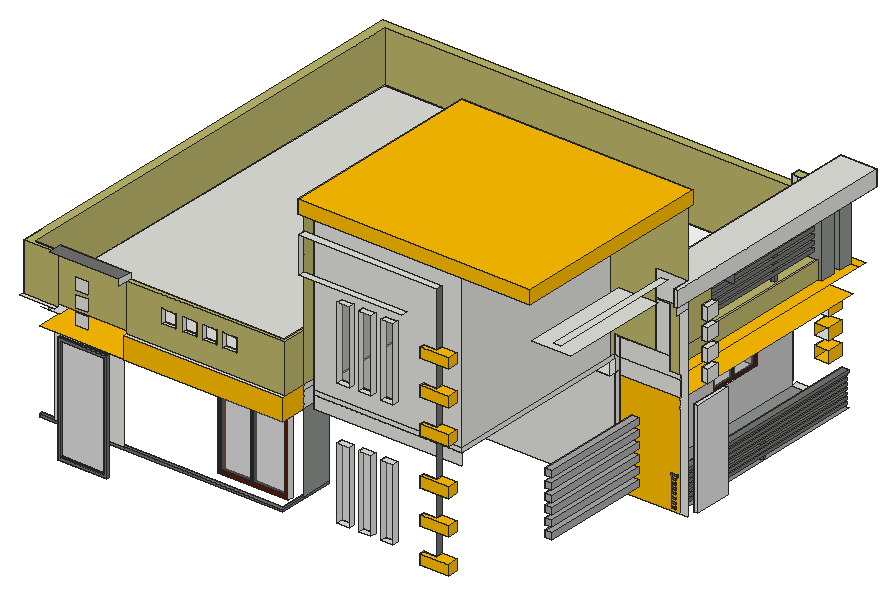
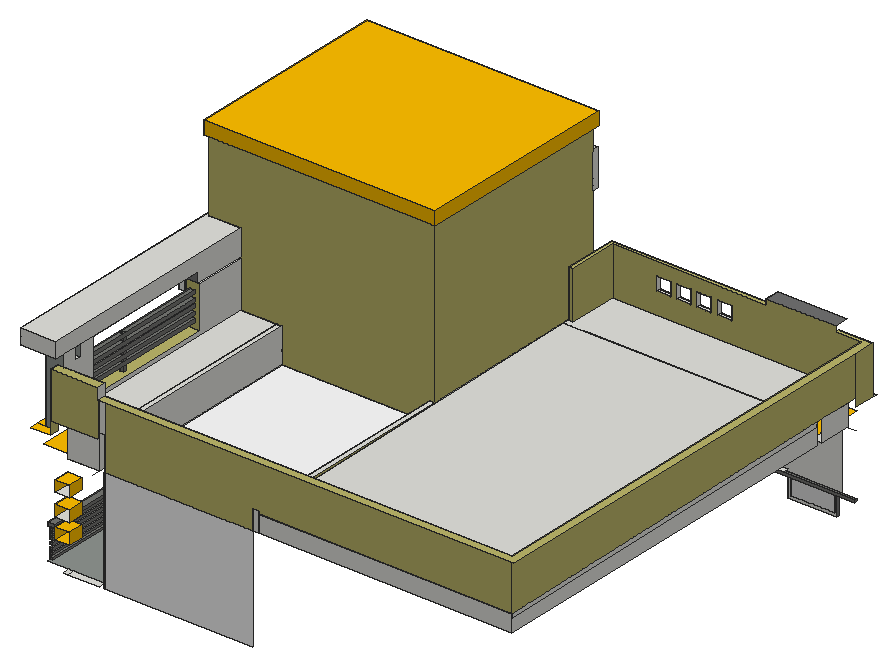
# SketchUp Ruby script. Lengths in inches.
U = 1.inch
M = Sketchup.active_model
def pt(a) = Geom::Point3d.new(a.map { |v| v * U })
def face(e, loops, mat)
  f = e.add_face(loops[0].map { |a| pt(a) })
  loops[1..].each { |l| e.add_face(l.map { |a| pt(a) }).erase! }
  f.material = f.back_material = mat if mat
  f
end
# faces: each face lists its corners as indices into pts; further lists are holes
def faces(e, pts, list, mat = nil) = list.each { |f| face(e, (f[0].is_a?(Array) ? f : [f]).map { |l| l.map { |i| pts[i] } }, mat) }
# xy, xz, yz: faces in a plane at the given z, y or x. An outline is a flat list of corners, or four numbers for a rectangle; further outlines are holes
def ring(l) = l.size == 4 ? [[l[0], l[1]], [l[2], l[1]], [l[2], l[3]], [l[0], l[3]]] : l.each_slice(2).to_a
def flat(e, list, mat, &to3) = list.each { |f| face(e, (f[0].is_a?(Array) ? f : [f]).map { |l| ring(l).map { |u, v| to3.(u, v) } }, mat) }
def xy(e, z, list, mat = nil) = flat(e, list, mat) { |x, y| [x, y, z] }
def xz(e, y, list, mat = nil) = flat(e, list, mat) { |x, z| [x, y, z] }
def yz(e, x, list, mat = nil) = flat(e, list, mat) { |y, z| [x, y, z] }
def lines(e, pts, list) = list.each { |a, b| e.add_line(pt(pts[a]), pt(pts[b])) }
# prism: a flat outline (further loops are holes) pulled along v
def prism(e, loops, v, mat = nil)
  f = face(e, loops, mat); d = Geom::Vector3d.new(v.map { |x| x * U })
  f.pushpull(f.normal.samedirection?(d) ? d.length : -d.length)
end
def box(e, o, s, mat = nil) = prism(e, [[o, [o[0] + s[0], o[1], o[2]], [o[0] + s[0], o[1] + s[1], o[2]], [o[0], o[1] + s[1], o[2]]]], [0, 0, s[2]], mat)
def at(x, y, z, deg = 0) = Geom::Transformation.translation(pt([x, y, z])) * Geom::Transformation.rotation(ORIGIN, Z_AXIS, deg.degrees)
def axes(o, x, y, z) = Geom::Transformation.new([*x, 0, *y, 0, *z, 0, *pt(o).to_a, 1])
def part(name) = M.definitions.add(name)
# library, detail: a bought-in or finely detailed component or shape, given as its bounding box
def library(name, o, s) = part(name).tap { |d| box(d.entities, o, s) }
def detail(e, o, s) = box(e.add_group.entities, o, s)
def put(e, d, t, mat = nil) = e.add_instance(d, t).tap { |i| i.material = mat if mat }
def group(e, t, mat = nil) = e.add_group.tap { |g| g.transformation = t; g.material = mat if mat }.entities
root = M.entities
M.materials.add("[0057_DarkKhaki]").color = [189, 183, 107]
M.materials.add("[0129_WhiteSmoke]").color = [245, 245, 245]
M.materials.add("[0132_LightGray]").color = [169, 169, 169]
M.materials.add("[Color B08]").color = [102, 25, 0]
M.materials.add("[Color D05]").color = [255, 191, 0]
M.materials.add("[Color M00]").color = [255, 255, 255]
M.materials.add("[Color M02]").color = [198, 198, 198]
M.materials.add("[Color M05]").color = [114, 114, 114]
M.materials.add("[Granite Light Gray]").color = [143, 148, 144]
M.materials.add("[Metal Seamed]").color = [118, 119, 115]
M.materials.add("[Stone Random Rubble]").color = [222, 222, 222]
M.materials.add("[Translucent Glass Gray]").color = [128, 128, 128]
M.materials["[Translucent Glass Gray]"].alpha = 0.5
c1 = part("Group\#2")
xy(c1.entities,0,[[0,0,52.875,0.9375],[0,0.9375,52.875,3.1875]],"[Color B08]")
xy(c1.entities,2.82,[[2.82,0,24.76,0.9375],[26.4375,0,50.05,0.9375],[2.82,0.9375,24.76,3.1875],[26.4375,0.9375,50.05,3.1875]],"[Color B08]")
xy(c1.entities,69.3,[[2.82,0,24.76,0.9375],[26.4375,0,50.05,0.9375],[2.82,0.9375,24.76,3.1875],[26.4375,0.9375,50.05,3.1875]],"[Color B08]")
xy(c1.entities,72.125,[[0,0,52.875,0.9375],[0,0.9375,52.875,3.1875]],"[Color B08]")
xz(c1.entities,0,[[[0,0,52.875,72.125],[26.4375,2.82,50.05,69.3],[2.82,2.82,24.76,69.3]]],"[Color B08]")
xz(c1.entities,0.9375,[[[0,0,52.875,72.125],[26.4375,2.82,50.05,69.3],[2.82,2.82,24.76,69.3]]],"[Color B08]")
xz(c1.entities,0.9375,[[2.82,2.82,24.76,69.3],[26.4375,2.82,50.05,69.3]],"[Translucent Glass Gray]")
xz(c1.entities,3.1875,[[[0,0,52.875,72.125],[26.4375,2.82,50.05,69.3],[2.82,2.82,24.76,69.3]]],"[Color B08]")
yz(c1.entities,0,[[0,0,0.9375,72.125],[0.9375,0,3.1875,72.125]],"[Color B08]")
yz(c1.entities,2.82,[[0,2.82,0.9375,69.3],[0.9375,2.82,3.1875,69.3]],"[Color B08]")
yz(c1.entities,24.76,[[0,2.82,0.9375,69.3],[0.9375,2.82,3.1875,69.3]],"[Color B08]")
yz(c1.entities,26.4375,[[0,2.82,0.9375,69.3],[0.9375,2.82,3.1875,69.3]],"[Color B08]")
yz(c1.entities,50.05,[[0,2.82,0.9375,69.3],[0.9375,2.82,3.1875,69.3]],"[Color B08]")
yz(c1.entities,52.875,[[0,0,0.9375,72.125],[0.9375,0,3.1875,72.125]],"[Color B08]")
c2 = part("Group\#1")
xy(c2.entities,0,[[0,0,48,3.0625]],"[Color B08]")
xy(c2.entities,3.38,[[3.38,0,12.79,3.0625],[12.79,0,14.23,3.0625],[14.23,0,44.62,3.0625]],"[Color B08]")
xy(c2.entities,80.62,[[3.38,0,12.79,3.0625],[12.79,0,14.23,3.0625],[14.23,0,44.62,3.0625]],"[Color B08]")
xy(c2.entities,84,[[0,0,48,3.0625]],"[Color B08]")
xz(c2.entities,0,[[[0,0,48,84],[3.38,3.38,44.62,80.62]]],"[Color B08]")
xz(c2.entities,1.4375,[[7.15,41.24,7.55,41.32,7.92,41.49,8.23,41.75,8.46,42.09,8.6,42.47,8.63,42.88,8.5625,43.28,8.39,43.65,8.125,43.96,7.79,44.19,7.4,44.33,7,44.37,6.6,44.29,6.23,44.12,5.92,43.86,5.68,43.52,5.55,43.14,5.51,42.73,5.59,42.33,5.76,41.96,6.02,41.65,6.36,41.42,6.74,41.28]],"[Metal Seamed]")
xz(c2.entities,3.0625,[[14.23,33.6,44.62,34.93]])
xz(c2.entities,3.0625,[[[0,0,48,84],[3.38,3.38,44.62,80.62]],[[3.38,3.38,12.79,80.62],[7.15,41.24,6.74,41.28,6.36,41.42,6.02,41.65,5.76,41.96,5.59,42.33,5.51,42.73,5.55,43.14,5.68,43.52,5.92,43.86,6.23,44.12,6.6,44.29,7,44.37,7.4,44.33,7.79,44.19,8.125,43.96,8.39,43.65,8.5625,43.28,8.63,42.88,8.6,42.47,8.46,42.09,8.23,41.75,7.92,41.49,7.55,41.32]],[14.23,3.38,44.62,10.1],[14.23,11.43,44.62,21.85],[14.23,23.18,44.62,33.6],
  [14.23,34.93,44.62,45.35],[14.23,46.68,44.62,57.1],[14.23,58.43,44.62,68.85],[14.23,70.18,44.62,80.62]],"[Color B08]")
xz(c2.entities,3.0625,[[12.79,3.38,14.23,3.38,14.23,10.1,44.62,10.1,44.62,11.43,14.23,11.43,14.23,21.85,44.62,21.85,44.62,23.18,14.23,23.18,14.23,45.35,44.62,45.35,44.62,46.68,14.23,46.68,14.23,57.1,44.62,57.1,44.62,58.43,14.23,58.43,14.23,68.85,44.62,68.85,44.62,70.18,14.23,70.18,14.23,80.62,12.79,80.62]],"[Color M00]")
xz(c2.entities,3.0625,[[7.15,41.24,6.74,41.28,6.36,41.42,6.02,41.65,5.76,41.96,5.59,42.33,5.51,42.73,5.55,43.14,5.68,43.52,5.92,43.86,6.23,44.12,6.6,44.29,7,44.37,7.4,44.33,7.79,44.19,8.125,43.96,8.39,43.65,8.5625,43.28,8.63,42.88,8.6,42.47,8.46,42.09,8.23,41.75,7.92,41.49,7.55,41.32]],"[Metal Seamed]")
yz(c2.entities,0,[[0,0,3.0625,84]],"[Color B08]")
yz(c2.entities,3.38,[[0,3.38,3.0625,80.62]],"[Color B08]")
yz(c2.entities,44.62,[[0,3.38,3.0625,80.62]],"[Color B08]")
yz(c2.entities,48,[[0,0,3.0625,84]],"[Color B08]")
p = [[6.74,3.0625,41.28],[7.15,3.0625,41.24],[7.15,1.4375,41.24],[6.74,1.4375,41.28],[7.55,3.0625,41.32],[7.55,1.4375,41.32],
  [6.36,3.0625,41.42],[6.36,1.4375,41.42],[7.92,3.0625,41.49],[7.92,1.4375,41.49],[6.02,3.0625,41.65],[6.02,1.4375,41.65],
  [8.23,3.0625,41.75],[8.23,1.4375,41.75],[5.76,3.0625,41.96],[5.76,1.4375,41.96],[8.46,3.0625,42.09],[8.46,1.4375,42.09],
  [5.59,3.0625,42.33],[5.59,1.4375,42.33],[8.6,3.0625,42.47],[8.6,1.4375,42.47],[5.51,3.0625,42.73],[5.51,1.4375,42.73],
  [8.63,3.0625,42.88],[8.63,1.4375,42.88],[5.55,3.0625,43.14],[5.55,1.4375,43.14],[8.5625,3.0625,43.28],[8.5625,1.4375,43.28],
  [5.68,3.0625,43.52],[5.68,1.4375,43.52],[8.39,3.0625,43.65],[8.39,1.4375,43.65],[5.92,3.0625,43.86],[5.92,1.4375,43.86],
  [8.125,3.0625,43.96],[8.125,1.4375,43.96],[6.23,3.0625,44.12],[6.23,1.4375,44.12],[7.79,3.0625,44.19],[7.79,1.4375,44.19],
  [6.6,3.0625,44.29],[6.6,1.4375,44.29],[7.4,3.0625,44.33],[7.4,1.4375,44.33],[7,3.0625,44.37],[7,1.4375,44.37]]
faces(c2.entities,p,[[0,1,2,3],[1,4,5,2],[6,0,3,7],[4,8,9,5],[10,6,7,11],[8,12,13,9],[14,10,11,15],[12,16,17,13],
  [18,14,15,19],[16,20,21,17],[22,18,19,23],[20,24,25,21],[26,22,23,27],[24,28,29,25],[30,26,27,31],[28,32,33,29],
  [34,30,31,35],[32,36,37,33],[38,34,35,39],[36,40,41,37],[42,38,39,43],[40,44,45,41],[46,42,43,47],[44,46,47,45]],"[Metal Seamed]")
box(root,[512.0625,256.47,332.9375],[6.0625,13.19,13.1875])
box(root,[512.0625,256.47,352.1875],[6.0625,13.19,13.1875])
box(root,[512.0625,256.47,371.4375],[6.0625,13.19,13.1875])
box(root,[512.0625,256.47,390.6875],[6.0625,13.19,13.1875])
xy(root,204.85,[[157.3,70.625,230.74,76.625]])
xy(root,207.96,[[45.85,2.375,96.92,4.6875]],"[Color M05]")
xy(root,210.78,[[48.67,2.375,94.1,4.6875]],"[Color M05]")
xy(root,211,[[432.3125,242.875,434.0625,274.21],[434.0625,274.21,438.3125,322.21],[432.3125,322.21,434.0625,472.9375],[438.3125,465.6875,471,472.9375],[471,465.6875,475.75,472.9375]])
xy(root,211,[[432.3125,274.21,434.0625,322.21]],"[Color M00]")
xy(root,211,[[[438.3125,242.875,498.1875,465.6875],[493.23,354.43,495.66,355.93],[493.23,357.31,495.66,358.81]]],"[Granite Light Gray]")
xy(root,211,[[493.23,354.43,495.66,355.93],[493.23,357.31,495.66,358.81]],"[Metal Seamed]")
xy(root,213.64,[[492.23,242.875,496.17,465.6875]],"[Metal Seamed]")
xy(root,216.08,[[492.23,242.875,496.17,465.6875]],"[Metal Seamed]")
xy(root,216.14,[[512.0625,246.21,516.3125,285.27]],"[Stone Random Rubble]")
xy(root,218.14,[[492.23,242.875,496.17,465.6875]],"[Metal Seamed]")
xy(root,220.58,[[492.23,242.875,496.17,465.6875]],"[Metal Seamed]")
xy(root,222.64,[[492.23,242.875,496.17,465.6875]],"[Metal Seamed]")
xy(root,224.54,[[403.14,26.875,403.14,31.1875,416.5625,31.1875,416.5625,38,432.5625,38,432.5625,26.875]])
xy(root,224.97,[[307.95,38,320.7,44],[330.08,38,342.83,44],[353.14,38,365.89,44]])
xy(root,225.08,[[492.23,242.875,496.17,465.6875]],"[Metal Seamed]")
xy(root,227.14,[[492.23,242.875,496.17,465.6875]],"[Metal Seamed]")
xy(root,229.58,[[492.23,242.875,496.17,465.6875]],"[Metal Seamed]")
xy(root,231.64,[[492.23,242.875,496.17,465.6875]],"[Metal Seamed]")
xy(root,234.08,[[492.23,242.875,496.17,465.6875]],"[Metal Seamed]")
xy(root,235,[[19.8125,10.9375,19.8125,14.6875,270.25,14.6875,270.25,70.625,273.0625,70.625,273.0625,10.9375]],"[Metal Seamed]")
xy(root,235.14,[[403.14,26.875,432.5625,26.875,432.5625,38,416.5625,38,416.5625,31.1875,403.14,31.1875]],"[Color D05]")
xy(root,236.14,[[492.23,242.875,496.17,465.6875]],"[Metal Seamed]")
xy(root,237.4375,[[19.8125,10.9375,273.0625,10.9375,273.0625,70.625,270.25,70.625,270.25,14.6875,19.8125,14.6875]],"[Metal Seamed]")
xy(root,238.58,[[492.23,242.875,496.17,465.6875]],"[Metal Seamed]")
xy(root,240.26,[[492.23,242.875,496.17,465.6875]],"[Metal Seamed]")
xy(root,240.5625,[[493.23,354.43,495.66,355.93]],"[Metal Seamed]")
xy(root,242.7,[[492.23,242.875,496.17,465.6875]],"[Metal Seamed]")
xy(root,243.89,[[[490.625,242.875,497.9375,465.6875],[493.23,357.31,495.66,358.81]]],"[Metal Seamed]")
xy(root,245.375,[[462.25,465.6875,477.19,481.9375]],"[Color D05]")
xy(root,247,[[490.625,242.875,497.9375,465.6875]],"[Metal Seamed]")
xy(root,248.59,[[432.3125,362.85,434.0625,422.35],[434.0625,362.85,438.3125,422.35]])
xy(root,255.96,[[488.42,82.3,495.55,195.3]],"[0132_LightGray]")
xy(root,257.3125,[[462.25,465.6875,477.19,481.9375]],"[Color D05]")
xy(root,260.54,[[403.14,26.875,403.14,31.1875,416.5625,31.1875,416.5625,38,432.5625,38,432.5625,26.875]])
xy(root,262.46,[[488.42,82.3,495.55,195.3]],"[0132_LightGray]")
xy(root,266.5,[[462.25,465.6875,477.19,481.9375]])
xy(root,267.52,[[488.42,82.3,495.55,195.3]],"[0132_LightGray]")
xy(root,271.14,[[403.14,26.875,432.5625,26.875,432.5625,38,416.5625,38,416.5625,31.1875,403.14,31.1875]],"[Color D05]")
xy(root,274.02,[[488.42,82.3,495.55,195.3]],"[0132_LightGray]")
xy(root,278.4375,[[462.25,465.6875,477.19,481.9375]],"[Color D05]")
xy(root,279.09,[[488.42,82.3,495.55,195.3]],"[0132_LightGray]")
xy(root,281.91,[[157.3,70.625,230.74,76.625]])
xy(root,283,[[43.95,70.625,91.95,76.625]])
xy(root,285.59,[[488.42,82.3,495.55,195.3]],"[0132_LightGray]")
xy(root,289.25,[[462.25,465.6875,477.19,481.9375]])
xy(root,290.65,[[488.42,82.3,495.55,195.3]],"[0132_LightGray]")
xy(root,292.66,[[432.3125,362.85,434.0625,422.35],[434.0625,362.85,438.3125,422.35]])
xy(root,295,[[432.3125,274.21,434.0625,322.21],[434.0625,274.21,438.3125,322.21]])
xy(root,296.54,[[403.14,26.875,403.14,31.1875,416.5625,31.1875,416.5625,38,432.5625,38,432.5625,26.875]],"[Color D05]")
xy(root,297.15,[[488.42,82.3,495.55,195.3]],"[0132_LightGray]")
xy(root,300.03,[[307.95,38,320.7,44],[330.08,38,342.83,44],[353.14,38,365.89,44]])
xy(root,301.1875,[[462.25,465.6875,477.19,481.9375]],"[Color D05]")
xy(root,302.21,[[488.42,82.3,495.55,195.3]],"[0132_LightGray]")
xy(root,307.14,[[403.14,26.875,432.5625,26.875,432.5625,38,416.5625,38,416.5625,31.1875,403.14,31.1875]],"[Color D05]")
xy(root,308.71,[[488.42,82.3,495.55,195.3]],"[0132_LightGray]")
xy(root,313.77,[[488.42,82.3,495.55,195.3]],"[0132_LightGray]")
xy(root,316.45,[[512.0625,246.21,516.3125,285.27]],"[Stone Random Rubble]")
xy(root,319,[[9,37.27,19.8125,70.625],[273.0625,76.625,279.0625,472.9375],[432.3125,242.875,434.0625,472.9375],[438.3125,465.6875,471,472.9375]])
xy(root,319,[[19.8125,10.9375,273.0625,70.625],[438.3125,242.875,502,465.6875]],"[Color D05]")
xy(root,319,[[279.0625,236.875,432.3125,242.875],[279.0625,242.875,432.3125,472.9375]],"[Color M00]")
xy(root,319.03,[[48.67,2.375,94.1,4.6875]])
xy(root,320.27,[[488.42,82.3,495.55,195.3]],"[0132_LightGray]")
xy(root,321.84,[[45.85,2.375,96.92,4.6875]],"[Color M05]")
xy(root,331.875,[[279.0625,44,432.3125,236.875]])
xy(root,336,[[279.0625,44,432.3125,236.875]])
xy(root,339.34,[[273.0625,242.875,279.0625,472.9375]])
xy(root,341,[[489.76,242.875,502,242.875,502,472.9375,493.64,472.9375,493.64,458.6875,481.39,458.6875,481.39,451.5,493.64,451.5,493.64,436,489.76,436],[481.39,472.9375,502,481.9375]],"[Color D05]")
xy(root,341.125,[[0,10.9375,35.5,15.25],[107.76,10.9375,273.0625,10.9375,273.0625,70.625,271.875,70.625,271.875,15.25,107.76,15.25],[9,19.25,267.875,19.25,267.875,70.625,273.0625,70.625,273.0625,76.625,9,76.625]])
xy(root,345.07,[[403.14,26.875,403.14,31.1875,416.5625,31.1875,416.5625,38,432.5625,38,432.5625,26.875]],"[Color D05]")
xy(root,354.75,[[432.3125,242.875,438.3125,472.9375],[438.3125,242.875,475,472.9375]])
xy(root,355.67,[[403.14,26.875,432.5625,26.875,432.5625,38,416.5625,38,416.5625,31.1875,403.14,31.1875]],"[Color D05]")
xy(root,355.72,[[307.95,38,320.7,44],[330.08,38,342.83,44],[353.14,38,365.89,44]])
xy(root,359.0625,[[[475,296.1875,487.01,436],[480.51,385.3,484.76,388.86]],[487.01,296.1875,489.76,436]],"[0057_DarkKhaki]")
xy(root,359.0625,[[480.51,385.3,484.76,388.86]],"[Metal Seamed]")
xy(root,363.22,[[143.89,15.25,158.45,19.25],[165.02,15.25,179.58,19.25],[186.14,15.25,200.7,19.25],[207.27,15.25,221.83,19.25]])
xy(root,365.4,[[480.01,293,485.33,436]],"[Metal Seamed]")
xy(root,369.09,[[480.01,293,485.33,436]],"[Metal Seamed]")
xy(root,371.78,[[480.01,291.5625,485.33,436]],"[Metal Seamed]")
xy(root,375.47,[[480.01,291.5625,485.33,436]],"[Metal Seamed]")
xy(root,377.79,[[143.89,15.25,158.45,19.25],[165.02,15.25,179.58,19.25],[186.14,15.25,200.7,19.25],[207.27,15.25,221.83,19.25]])
xy(root,378.15,[[480.01,296.1875,485.33,436]],"[Metal Seamed]")
xy(root,381.07,[[403.14,26.875,403.14,31.1875,416.5625,31.1875,416.5625,38,432.5625,38,432.5625,26.875]],"[Color D05]")
xy(root,381.84,[[480.01,296.1875,485.33,436]],"[Metal Seamed]")
xy(root,384.47,[[480.01,296,485.33,436]],"[Metal Seamed]")
xy(root,388.15,[[480.01,296,485.33,436]],"[Metal Seamed]")
xy(root,390.75,[[0,15.25,35.5,15.25,35.5,19.25,9,19.25,9,472.9375,432.3125,472.9375,432.3125,481.9375,0,481.9375],[107.76,15.25,271.875,15.25,271.875,70.625,267.875,70.625,267.875,19.25,107.76,19.25]],"[0057_DarkKhaki]")
xy(root,391.34,[[480.01,296.1875,485.33,436]],"[Metal Seamed]")
xy(root,391.67,[[403.14,26.875,432.5625,26.875,432.5625,38,416.5625,38,416.5625,31.1875,403.14,31.1875]],"[Color D05]")
xy(root,395.03,[[480.01,296.1875,485.33,436],[480.51,385.3,484.76,388.86]],"[Metal Seamed]")
xy(root,396.4375,[[35.5,4.6875,107.76,19.25]],"[Color M05]")
xy(root,402.75,[[475,242.875,489.76,296.1875],[475,451.5,481.39,458.6875]])
xy(root,402.75,[[432.3125,472.9375,481.39,481.9375]],"[0057_DarkKhaki]")
xy(root,404.84,[[475,242.875,500.3125,298.6875]])
xy(root,414.75,[[508.125,225.38,512.0625,228.57],[475,298.6875,475,436,493.64,436,493.64,451.5,475,451.5,475,458.6875,493.64,458.6875,493.64,472.9375,475,472.9375,475,483.5625,512.0625,483.5625,512.0625,298.6875],[475,436,493.64,451.5],[475,458.6875,493.64,472.9375]])
xy(root,417.07,[[403.14,26.875,403.14,31.1875,416.5625,31.1875,416.5625,38,432.5625,38,432.5625,26.875]],"[Color D05]")
xy(root,427.67,[[403.14,26.875,432.5625,26.875,432.5625,38,416.5625,38,416.5625,31.1875,403.14,31.1875]],"[Color D05]")
xy(root,430.78,[[307.95,38,320.7,44],[330.08,38,342.83,44],[353.14,38,365.89,44]])
xy(root,431.25,[[508.125,225.38,512.0625,225.38,512.0625,483.5625,475,483.5625,475,242.875,508.125,242.875]])
xy(root,433.9,[[474.9375,82.3,515.125,195.3]])
xy(root,447.125,[[273.0625,31.1875,380.5625,38]])
xy(root,449.28,[[508.125,69.42,515.125,208.18]])
xy(root,484.625,[[273.0625,31.1875,416.5625,38]])
xy(root,504.125,[[446.125,34.9375,450.58,38],[462.0625,34.9375,466.51,38],[478.1875,34.9375,482.64,38],[273.0625,38,508.125,242.875]])
xy(root,504.125,[[273.0625,30.0625,273.0625,38,446.125,38,446.125,34.9375,450.58,34.9375,450.58,38,462.0625,38,462.0625,34.9375,466.51,34.9375,466.51,38,478.1875,38,478.1875,34.9375,482.64,34.9375,482.64,38,508.125,38,508.125,242.875,514.1875,242.875,514.1875,30.0625]],"[Color D05]")
xy(root,507.625,[[279.0625,44,432.3125,236.875]])
xy(root,517.9375,[[273.0625,30.0625,514.1875,242.875]],"[Color D05]")
xz(root,2.375,[[[45.85,207.96,96.92,321.84],[48.67,210.78,94.1,319.03]]],"[Color M05]")
xz(root,4.6875,[[[45.85,207.96,96.92,321.84],[48.67,210.78,94.1,319.03]],[63.1875,338.16,75.3125,350.29],[63.1875,354.54,75.3125,366.66],[63.1875,370.91,75.3125,383.04]])
xz(root,4.6875,[[48.67,210.78,94.1,319.03]],"[Stone Random Rubble]")
xz(root,10.9375,[[35.5,237.4375,107.76,319]])
xz(root,10.9375,[[107.76,319,273.0625,341.125]],"[Color D05]")
xz(root,10.9375,[[19.8125,235,35.5,237.4375],[35.5,235,107.76,237.4375],[107.76,235,273.0625,237.4375]],"[Metal Seamed]")
xz(root,14.6875,[[19.8125,235,270.25,237.4375]],"[Metal Seamed]")
xz(root,15.25,[[0,341.125,35.5,390.75],[[107.76,341.125,271.875,390.75],[143.89,363.22,158.45,377.79],[165.02,363.22,179.58,377.79],[186.14,363.22,200.7,377.79],[207.27,363.22,221.83,377.79]]],"[0057_DarkKhaki]")
xz(root,19.25,[[[9,341.125,9,390.75,35.5,390.75,35.5,396.4375,107.76,396.4375,107.76,390.75,267.875,390.75,267.875,341.125],[143.89,363.22,158.45,377.79],[165.02,363.22,179.58,377.79],[186.14,363.22,200.7,377.79],[207.27,363.22,221.83,377.79]]],"[0057_DarkKhaki]")
xz(root,26.875,[[403.14,224.54,432.5625,235.14],[403.14,260.54,432.5625,271.14],[403.14,296.54,432.5625,307.14],[403.14,345.07,432.5625,355.67],[403.14,381.07,432.5625,391.67],
  [403.14,417.07,432.5625,427.67]],"[Color D05]")
xz(root,30.0625,[[273.0625,504.125,514.1875,517.9375]],"[Color D05]")
xz(root,31.1875,[[403.14,224.54,416.5625,235.14],[403.14,260.54,416.5625,271.14],[403.14,296.54,416.5625,307.14],[403.14,345.07,416.5625,355.67],[403.14,381.07,416.5625,391.67],
  [403.14,417.07,416.5625,427.67]])
xz(root,44,[[279.0625,319,432.3125,331.875],[279.0625,331.875,432.3125,336],[[279.0625,336,432.3125,507.625],[307.95,355.72,320.7,430.78],[330.08,355.72,342.83,430.78],[353.14,355.72,365.89,430.78]]])
xz(root,44,[[307.95,224.97,320.7,300.03],[330.08,224.97,342.83,300.03],[353.14,224.97,365.89,300.03],[307.95,355.72,320.7,430.78],[330.08,355.72,342.83,430.78],
  [353.14,355.72,365.89,430.78]],"[Translucent Glass Gray]")
xz(root,70.625,[[267.875,341.125,271.875,390.75]],"[0057_DarkKhaki]")
xz(root,70.625,[[270.25,235,273.0625,237.4375]],"[Metal Seamed]")
xz(root,76.625,[[9,319,273.0625,341.125]])
xz(root,82.3,[[488.42,255.96,495.55,262.46],[488.42,267.52,495.55,274.02],[488.42,279.09,495.55,285.59],[488.42,290.65,495.55,297.15],[488.42,302.21,495.55,308.71],
  [488.42,313.77,495.55,320.27]],"[0132_LightGray]")
xz(root,225.38,[[508.125,414.75,512.0625,431.25]])
xz(root,236.875,[[279.0625,336,432.3125,507.625]])
xz(root,236.875,[[279.0625,319,432.3125,331.875]],"[Color M00]")
xz(root,242.875,[[279.0625,211,432.3125,319],[432.3125,211,434.0625,319],[500.3125,211,508.125,211,508.125,404.84,500.3125,404.84,500.3125,341,502,341,502,319,500.3125,319],[438.3125,319,500.3125,336],[500.3125,319,502,336],
  [432.3125,336,438.3125,354.75],[438.3125,336,438.3125,354.75,489.76,354.75,489.76,341,500.3125,341,500.3125,336],[500.3125,336,502,341],[475,354.75,489.76,402.75],[475,404.84,508.125,431.25]])
xz(root,242.875,[[279.0625,319,279.0625,339.34,273.0625,339.34,273.0625,504.125,508.125,504.125,508.125,431.25,475,431.25,475,404.84,500.3125,404.84,500.3125,341,489.76,341,489.76,402.75,475,402.75,475,354.75,432.3125,354.75,432.3125,319]],"[0057_DarkKhaki]")
xz(root,242.875,[[[438.3125,211,500.3125,319],[490.625,243.89,497.9375,247],[492.23,227.14,496.17,229.58],[492.23,218.14,496.17,220.58],[492.23,213.64,496.17,216.08],[492.23,222.64,496.17,225.08],[492.23,231.64,496.17,234.08],[492.23,236.14,496.17,238.58],[492.23,240.26,496.17,242.7]],[273.0625,504.125,514.1875,517.9375]],"[Color D05]")
xz(root,246.21,[[512.0625,216.14,516.3125,316.45]],"[Stone Random Rubble]")
xz(root,274.21,[[432.3125,211,434.0625,295],[434.0625,211,438.3125,295]])
xz(root,285.27,[[512.0625,216.14,516.3125,316.45]],"[Stone Random Rubble]")
xz(root,291.5625,[[480.01,371.78,485.33,375.47]],"[Metal Seamed]")
xz(root,293,[[480.01,365.4,485.33,369.09]],"[Metal Seamed]")
xz(root,296,[[480.01,384.47,485.33,388.15]],"[Metal Seamed]")
xz(root,296.1875,[[[475,359.0625,489.76,402.75],[480.01,391.34,485.33,395.03],[480.01,378.15,485.33,381.84]]],"[0057_DarkKhaki]")
xz(root,298.6875,[[475,404.84,512.0625,414.75]],"[Color M05]")
xz(root,322.21,[[432.3125,211,434.0625,295],[434.0625,211,438.3125,295]])
xz(root,354.43,[[493.23,211,495.66,240.5625]],"[Metal Seamed]")
xz(root,355.93,[[493.23,211,495.66,240.5625]],"[Metal Seamed]")
xz(root,357.31,[[493.23,211,495.66,243.89]],"[Metal Seamed]")
xz(root,358.81,[[493.23,211,495.66,243.89]],"[Metal Seamed]")
xz(root,362.85,[[432.3125,248.59,434.0625,292.66],[434.0625,248.59,438.3125,292.66]])
xz(root,385.3,[[480.51,359.0625,484.76,395.03]],"[Metal Seamed]")
xz(root,388.86,[[480.51,359.0625,484.76,395.03]],"[Metal Seamed]")
xz(root,422.35,[[432.3125,248.59,434.0625,292.66],[434.0625,248.59,438.3125,292.66]])
xz(root,436,[[[489.76,341,493.64,341,493.64,414.75,475,414.75,475,359.0625,489.76,359.0625],[480.01,365.4,485.33,369.09],[480.01,371.78,485.33,375.47],[480.01,378.15,485.33,381.84],[480.01,384.47,485.33,388.15],[480.01,391.34,485.33,395.03]]],"[Granite Light Gray]")
xz(root,436,[[480.01,365.4,485.33,369.09],[480.01,371.78,485.33,375.47],[480.01,378.15,485.33,381.84],[480.01,384.47,485.33,388.15],[480.01,391.34,485.33,395.03]],"[Metal Seamed]")
xz(root,451.5,[[481.39,341,481.39,402.75,475,402.75,475,414.75,493.64,414.75,493.64,341]],"[Granite Light Gray]")
xz(root,458.6875,[[481.39,341,493.64,341,493.64,414.75,475,414.75,475,402.75,481.39,402.75]],"[Granite Light Gray]")
xz(root,465.6875,[[492.23,213.64,496.17,216.08],[492.23,218.14,496.17,220.58],[492.23,222.64,496.17,225.08],[492.23,227.14,496.17,229.58],[492.23,231.64,496.17,234.08],
  [492.23,236.14,496.17,238.58],[492.23,240.26,496.17,242.7],[490.625,243.89,497.9375,247]],"[Metal Seamed]")
xz(root,472.9375,[[432.3125,211,434.0625,319],[9,319,273.0625,336.875],[273.0625,319,279.0625,339.34],[438.3125,319,471,354.75],[432.3125,354.75,438.3125,402.75],
  [438.3125,354.75,471,402.75],[471,354.75,475,402.75]])
xz(root,472.9375,[[279.0625,319,432.3125,319,432.3125,390.75,9,390.75,9,336.875,273.0625,336.875,273.0625,339.34,279.0625,339.34]],"[0057_DarkKhaki]")
xz(root,472.9375,[[279.0625,211,432.3125,319]],"[0129_WhiteSmoke]")
xz(root,472.9375,[[481.39,341,481.39,402.75,475,402.75,475,414.75,493.64,414.75,493.64,341]],"[Granite Light Gray]")
xz(root,481.9375,[[432.3125,354.75,481.39,402.75]],"[0057_DarkKhaki]")
xz(root,483.5625,[[475,414.75,512.0625,431.25]])
yz(root,0,[[15.25,341.125,37.27,390.75]],"[0057_DarkKhaki]")
yz(root,9,[[37.27,319,70.625,341.125],[76.625,319,472.9375,319,472.9375,336.875,472.88,331.4375,76.625,335.6875],[472.88,331.4375,472.9375,336.875,76.625,341.125,76.625,335.6875],[76.57,335.6875,76.625,341.125,76.625,335.6875]])
yz(root,9,[[472.9375,336.875,472.9375,390.75,19.25,390.75,19.25,341.125,76.625,341.125]],"[0057_DarkKhaki]")
yz(root,19.8125,[[10.9375,235,14.6875,237.4375]],"[Metal Seamed]")
yz(root,45.85,[[2.375,207.96,4.6875,321.84]],"[Color M05]")
yz(root,48.67,[[2.375,210.78,4.6875,319.03]],"[Color M05]")
yz(root,94.1,[[2.375,210.78,4.6875,319.03]],"[Color M05]")
yz(root,96.92,[[2.375,207.96,4.6875,321.84]],"[Color M05]")
yz(root,107.76,[[4.6875,390.75,19.25,396.4375]])
yz(root,143.89,[[15.25,363.22,19.25,377.79]])
yz(root,157.3,[[70.625,204.85,76.625,281.91]])
yz(root,158.45,[[15.25,363.22,19.25,377.79]])
yz(root,165.02,[[15.25,363.22,19.25,377.79]])
yz(root,179.58,[[15.25,363.22,19.25,377.79]])
yz(root,186.14,[[15.25,363.22,19.25,377.79]])
yz(root,200.7,[[15.25,363.22,19.25,377.79]])
yz(root,207.27,[[15.25,363.22,19.25,377.79]])
yz(root,221.83,[[15.25,363.22,19.25,377.79]])
yz(root,230.74,[[70.625,204.85,76.625,281.91]])
yz(root,267.875,[[19.25,341.125,70.625,390.75]],"[0057_DarkKhaki]")
yz(root,270.25,[[14.6875,235,70.625,237.4375]],"[Metal Seamed]")
yz(root,271.875,[[15.25,341.125,70.625,390.75]],"[0057_DarkKhaki]")
yz(root,273.0625,[[38,319,70.625,336],[76.625,319,76.625,335.6875,242.82,333.9,472.88,331.4375,472.9375,336.875,472.9375,319],[472.88,331.4375,242.82,333.9,242.875,339.34,472.9375,336.875],[242.82,333.9,242.875,339.34,76.625,341.125,76.625,335.6875],[76.57,335.6875,76.625,336],
  [38,336,70.625,341.125],[70.625,336,70.625,341.125,76.625,341.125,76.57,336],[76.57,336,76.625,341.125,76.625,336],[31.1875,447.125,38,484.625]])
yz(root,273.0625,[[472.9375,336.875,242.875,339.34,76.625,341.125,38,341.125,38,504.125,242.875,504.125,242.875,339.34,472.9375,339.34]],"[0057_DarkKhaki]")
yz(root,273.0625,[[10.9375,319,38,341.125],[30.0625,504.125,242.875,517.9375]],"[Color D05]")
yz(root,273.0625,[[38,237.4375,70.625,319]],"[Granite Light Gray]")
yz(root,273.0625,[[10.9375,235,38,237.4375],[38,235,70.625,237.4375]],"[Metal Seamed]")
yz(root,279.0625,[[44,319,236.875,331.875],[242.875,319,472.9375,339.34],[44,331.875,242.875,336],[44,336,236.875,507.625]])
yz(root,279.0625,[[236.875,319,242.875,331.875]],"[Color M00]")
yz(root,307.95,[[38,224.97,44,300.03],[38,355.72,44,430.78]])
yz(root,320.7,[[38,224.97,44,300.03],[38,355.72,44,430.78]])
yz(root,330.08,[[38,224.97,44,300.03],[38,355.72,44,430.78]])
yz(root,342.83,[[38,224.97,44,300.03],[38,355.72,44,430.78]])
yz(root,353.14,[[38,224.97,44,300.03],[38,355.72,44,430.78]])
yz(root,365.89,[[38,224.97,44,300.03],[38,355.72,44,430.78]])
yz(root,403.14,[[26.875,224.54,31.1875,235.14],[26.875,260.54,31.1875,271.14],[26.875,296.54,31.1875,307.14],[26.875,345.07,31.1875,355.67],[26.875,381.07,31.1875,391.67],
  [26.875,417.07,31.1875,427.67]],"[Color D05]")
yz(root,416.5625,[[31.1875,224.54,38,235.14],[31.1875,260.54,38,271.14],[31.1875,296.54,38,307.14],[31.1875,345.07,38,355.67],[31.1875,381.07,38,391.67],
  [31.1875,417.07,38,427.67]])
yz(root,416.5625,[[31.1875,235.14,38,260.54],[31.1875,271.14,38,296.54],[31.1875,307.14,38,345.07],[31.1875,355.67,38,381.07],[31.1875,391.67,38,417.07],
  [31.1875,427.67,38,484.625]],"[Color M05]")
yz(root,432.3125,[[[242.875,211,242.875,319,472.9375,319,472.9375,211,322.21,211,322.21,295,274.21,295,274.21,211],[362.85,248.59,422.35,292.66]],[242.875,319,472.9375,354.75],[44,331.875,242.875,336],[44,336,236.875,507.625],[472.9375,390.75,481.9375,402.75]])
yz(root,432.3125,[[236.875,319,242.875,331.875]],"[Color M00]")
yz(root,432.5625,[[26.875,224.54,38,235.14],[26.875,260.54,38,271.14],[26.875,296.54,38,307.14],[26.875,345.07,38,355.67],[26.875,381.07,38,391.67],
  [26.875,417.07,38,427.67]],"[Color D05]")
yz(root,434.0625,[[[242.875,211,274.21,211,274.21,295,322.21,295,322.21,211,472.9375,211,472.9375,319,242.875,319],[362.85,248.59,422.35,292.66]]])
yz(root,438.3125,[[242.875,319,472.9375,354.75]])
yz(root,438.3125,[[[242.875,211,274.21,211,274.21,295,322.21,295,322.21,211,465.6875,211,465.6875,319,242.875,319],[362.85,248.59,422.35,292.66]]],"[Color M02]")
yz(root,462.25,[[465.6875,245.375,481.9375,257.3125],[465.6875,266.5,481.9375,278.4375],[465.6875,289.25,481.9375,301.1875]],"[Color D05]")
yz(root,475,[[242.875,354.75,242.875,402.75,296.1875,402.75,296.1875,359.0625,436,359.0625,436,414.75,451.5,414.75,451.5,402.75,458.6875,402.75,458.6875,414.75,472.9375,414.75,472.9375,354.75],[242.875,404.84,242.875,431.25,483.5625,431.25,483.5625,414.75,298.6875,414.75,298.6875,404.84]])
yz(root,477.19,[[465.6875,245.375,481.9375,257.3125],[465.6875,266.5,481.9375,278.4375],[465.6875,289.25,481.9375,301.1875]],"[Color D05]")
yz(root,480.01,[[293,365.4,436,369.09],[291.5625,371.78,436,375.47],[296.1875,378.15,436,381.84],[296,384.47,436,388.15],[296.1875,391.34,436,395.03]],"[Metal Seamed]")
yz(root,480.51,[[385.3,359.0625,388.86,395.03]],"[Metal Seamed]")
yz(root,481.39,[[451.5,341,458.6875,402.75],[472.9375,341,481.9375,402.75]],"[0057_DarkKhaki]")
yz(root,484.76,[[385.3,359.0625,388.86,395.03]],"[Metal Seamed]")
yz(root,485.33,[[293,365.4,436,369.09],[291.5625,371.78,436,375.47],[296.1875,378.15,436,381.84],[296,384.47,436,388.15],[296.1875,391.34,436,395.03]],"[Metal Seamed]")
yz(root,488.42,[[82.3,255.96,195.3,262.46],[82.3,267.52,195.3,274.02],[82.3,279.09,195.3,285.59],[82.3,290.65,195.3,297.15],[82.3,302.21,195.3,308.71],
  [82.3,313.77,195.3,320.27]],"[0132_LightGray]")
yz(root,489.76,[[242.875,341,296.1875,354.75],[296.1875,341,436,359.0625],[242.875,354.75,296.1875,402.75]],"[0057_DarkKhaki]")
yz(root,490.625,[[242.875,243.89,465.6875,247]],"[Metal Seamed]")
yz(root,492.23,[[242.875,213.64,465.6875,216.08],[242.875,218.14,465.6875,220.58],[242.875,222.64,465.6875,225.08],[242.875,227.14,465.6875,229.58],[242.875,231.64,465.6875,234.08],
  [242.875,236.14,465.6875,238.58],[242.875,240.26,465.6875,242.7]],"[Metal Seamed]")
yz(root,493.23,[[354.43,211,355.93,240.5625],[357.31,211,358.81,243.89]],"[Metal Seamed]")
yz(root,493.64,[[436,341,451.5,414.75],[458.6875,341,472.9375,414.75]],"[Granite Light Gray]")
yz(root,495.55,[[82.3,255.96,195.3,262.46],[82.3,267.52,195.3,274.02],[82.3,279.09,195.3,285.59],[82.3,290.65,195.3,297.15],[82.3,302.21,195.3,308.71],
  [82.3,313.77,195.3,320.27]],"[0132_LightGray]")
yz(root,495.66,[[354.43,211,355.93,240.5625],[357.31,211,358.81,243.89]],"[Metal Seamed]")
yz(root,496.17,[[242.875,213.64,465.6875,216.08],[242.875,218.14,465.6875,220.58],[242.875,222.64,465.6875,225.08],[242.875,227.14,465.6875,229.58],[242.875,231.64,465.6875,234.08],
  [242.875,236.14,465.6875,238.58],[242.875,240.26,465.6875,242.7]],"[Metal Seamed]")
yz(root,497.9375,[[242.875,243.89,465.6875,247]],"[Metal Seamed]")
yz(root,508.125,[[228.57,404.84,242.875,404.84,242.875,431.25,225.38,431.25,225.38,414.75,228.57,414.75]])
yz(root,512.0625,[[246.21,216.14,285.27,316.45],[225.38,414.75,483.5625,431.25]])
yz(root,514.1875,[[30.0625,504.125,242.875,517.9375]],"[Color D05]")
yz(root,516.3125,[[246.21,216.14,285.27,316.45]],"[Stone Random Rubble]")
p = [[9,76.625,335.6875],[9,472.88,331.4375],[273.0625,472.88,331.4375],[273.0625,242.82,333.9],[273.0625,76.625,335.6875],[273.0625,76.57,335.6875],
  [254.48,76.57,335.6875],[248.5625,76.57,335.6875],[9,76.57,335.6875],[9,472.9375,336.875],[273.0625,472.9375,336.875],[248.5625,76.625,341.125],
  [9,76.625,341.125],[254.48,76.625,341.125],[273.0625,76.625,341.125],[273.0625,76.57,336],[273.0625,242.875,339.34],[279.0625,242.875,336],
  [273.0625,242.875,336],[9,37.27,319],[0,37.27,319],[438.3125,472.9375,319],[438.3125,481.9375,319],[279.0625,57,512.625],
  [279.0625,57,507.625],[432.3125,236.875,507.625],[432.3125,236.875,512.625],[432.3125,44,507.625],[432.3125,44,512.625],[279.0625,44,507.625],
  [279.0625,44,512.625]]
faces(root,p,[[0,1,2,3,4,5,6,7,8],[9,10,2,1],[11,12,8,7],[13,11,7,6],[14,13,6,5,15],[9,12,11,13,14,16,10]])
lines(root,p,[[17,18],[19,20],[21,22],[23,24],[25,26],[27,28],[29,30]])
put(root,c1,axes([157.3,70.625,204.85],[1.38889,0,0],[0,1.405,0],[0,0,1.06846]))
put(root,c2,at(438.3125,274.21,211,90))
put(root,c1,axes([436.94,362.85,248.59],[0,1.1253,0],[-0.90125,0,0],[0,0,0.61092]))
